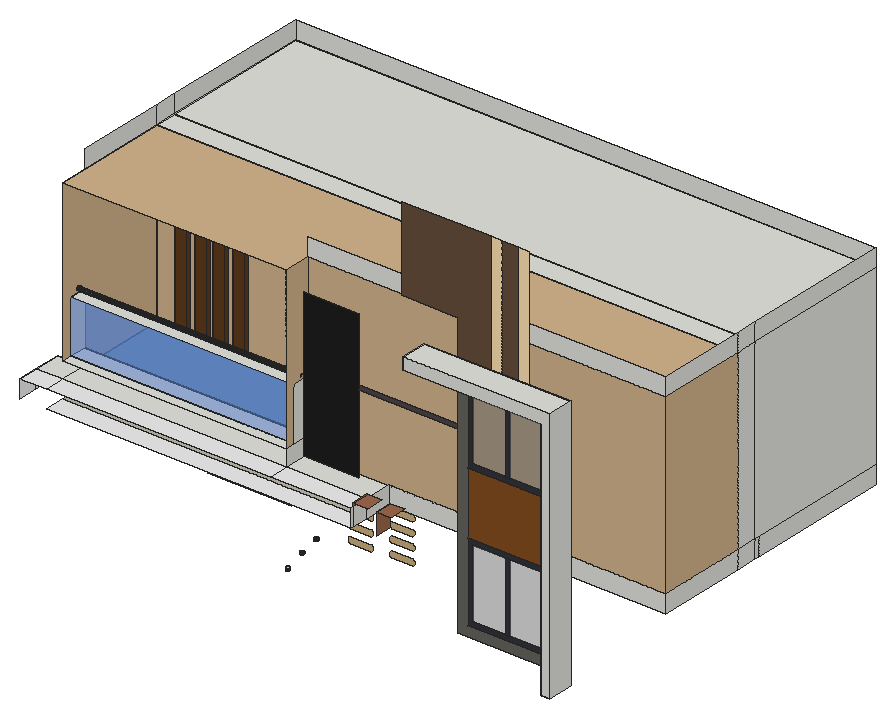
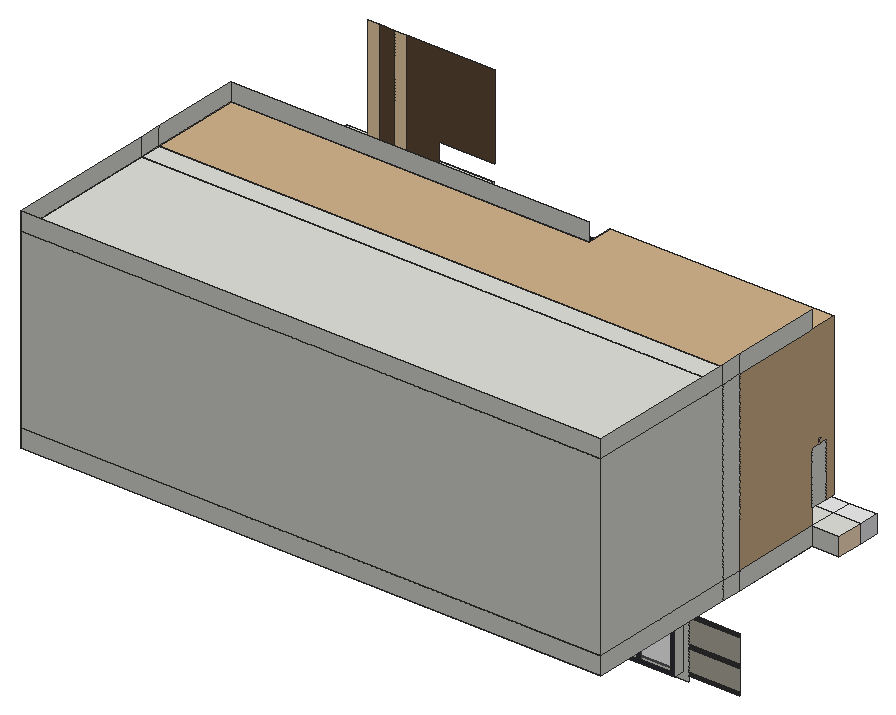
# SketchUp Ruby script. Lengths in inches.
U = 1.inch
M = Sketchup.active_model
def pt(a) = Geom::Point3d.new(a.map { |v| v * U })
def face(e, loops, mat)
  f = e.add_face(loops[0].map { |a| pt(a) })
  loops[1..].each { |l| e.add_face(l.map { |a| pt(a) }).erase! }
  f.material = f.back_material = mat if mat
  f
end
# faces: each face lists its corners as indices into pts; further lists are holes
def faces(e, pts, list, mat = nil) = list.each { |f| face(e, (f[0].is_a?(Array) ? f : [f]).map { |l| l.map { |i| pts[i] } }, mat) }
# xy, xz, yz: faces in a plane at the given z, y or x. An outline is a flat list of corners, or four numbers for a rectangle; further outlines are holes
def ring(l) = l.size == 4 ? [[l[0], l[1]], [l[2], l[1]], [l[2], l[3]], [l[0], l[3]]] : l.each_slice(2).to_a
def flat(e, list, mat, &to3) = list.each { |f| face(e, (f[0].is_a?(Array) ? f : [f]).map { |l| ring(l).map { |u, v| to3.(u, v) } }, mat) }
def xy(e, z, list, mat = nil) = flat(e, list, mat) { |x, y| [x, y, z] }
def xz(e, y, list, mat = nil) = flat(e, list, mat) { |x, z| [x, y, z] }
def yz(e, x, list, mat = nil) = flat(e, list, mat) { |y, z| [x, y, z] }
def lines(e, pts, list) = list.each { |a, b| e.add_line(pt(pts[a]), pt(pts[b])) }
# prism: a flat outline (further loops are holes) pulled along v
def prism(e, loops, v, mat = nil)
  f = face(e, loops, mat); d = Geom::Vector3d.new(v.map { |x| x * U })
  f.pushpull(f.normal.samedirection?(d) ? d.length : -d.length)
end
def box(e, o, s, mat = nil) = prism(e, [[o, [o[0] + s[0], o[1], o[2]], [o[0] + s[0], o[1] + s[1], o[2]], [o[0], o[1] + s[1], o[2]]]], [0, 0, s[2]], mat)
def at(x, y, z, deg = 0) = Geom::Transformation.translation(pt([x, y, z])) * Geom::Transformation.rotation(ORIGIN, Z_AXIS, deg.degrees)
def axes(o, x, y, z) = Geom::Transformation.new([*x, 0, *y, 0, *z, 0, *pt(o).to_a, 1])
def part(name) = M.definitions.add(name)
# library, detail: a bought-in or finely detailed component or shape, given as its bounding box
def library(name, o, s) = part(name).tap { |d| box(d.entities, o, s) }
def detail(e, o, s) = box(e.add_group.entities, o, s)
def put(e, d, t, mat = nil) = e.add_instance(d, t).tap { |i| i.material = mat if mat }
def group(e, t, mat = nil) = e.add_group.tap { |g| g.transformation = t; g.material = mat if mat }.entities
root = M.entities
M.materials.add("[0012_Bisque]").color = [255, 228, 196]
M.materials.add("[0035_Tan]").color = [210, 180, 140]
M.materials.add("[Asphalt New]").color = [79, 70, 73]
M.materials.add("[Blacktop New]").color = [30, 30, 30]
M.materials.add("[Blinds Vertical Pattern]").color = [237, 237, 239]
M.materials.add("[Carrera Marble]").color = [207, 207, 207]
M.materials.add("[Cladding Siding Tan]").color = [102, 79, 59]
M.materials.add("[Color M07]").color = [58, 58, 58]
M.materials.add("[Concrete Pavers Block Multi]").color = [124, 140, 145]
M.materials.add("[Formica Beige]").color = [255, 225, 180]
M.materials.add("[Formica Graystone]").color = [91, 89, 83]
M.materials.add("[Formica Graystone]1").color = [188, 184, 170]
M.materials.add("[Formica Graystone]2").color = [102, 99, 92]
M.materials.add("[Formica Laminate Dark]").color = [50, 53, 60]
M.materials.add("[Formica Speckled Grey]").color = [94, 105, 111]
M.materials.add("[Quartz Light Grey]").color = [251, 251, 252]
M.materials.add("[Translucent Glass Blue]").color = [106, 158, 252]
M.materials["[Translucent Glass Blue]"].alpha = 0.5
M.materials.add("[Translucent Glass Gray]").color = [128, 128, 128]
M.materials["[Translucent Glass Gray]"].alpha = 0.5
M.materials.add("[Wood Bamboo]").color = [130, 77, 31]
M.materials.add("[Wood Floor Light]").color = [204, 176, 127]
M.materials.add("[Wood Floor Parquet]").color = [96, 59, 26]
M.materials.add("[Wood Veneer 02]").color = [155, 104, 74]
prism(root,[[[158.39,214.66,43.5],[158.09,214.43,43.5],[157.74,214.28,43.5],[157.37,214.23,43.5],[157,214.28,43.5],[156.65,214.43,43.5],[156.35,214.66,43.5],[156.125,214.95,43.5],[155.98,215.3,43.5],[155.93,215.67,43.5],[155.98,216.04,43.5],[156.125,216.39,43.5],[156.35,216.6875,43.5],[156.65,216.92,43.5],[157,217.0625,43.5],[157.37,217.11,43.5],[157.74,217.0625,43.5],[158.09,216.92,43.5],[158.39,216.6875,43.5],[158.62,216.39,43.5],[158.76,216.04,43.5],[158.81,215.67,43.5],[158.76,215.3,43.5],[158.62,214.95,43.5]]],[0,0,1.5625])
prism(root,[[[157.57,229.04,47.875],[157.28,228.81,47.875],[156.93,228.66,47.875],[156.56,228.62,47.875],[156.1875,228.66,47.875],[155.84,228.81,47.875],[155.54,229.04,47.875],[155.3125,229.33,47.875],[155.17,229.68,47.875],[155.12,230.05,47.875],[155.17,230.43,47.875],[155.3125,230.77,47.875],[155.54,231.07,47.875],[155.84,231.3,47.875],[156.1875,231.44,47.875],[156.56,231.49,47.875],[156.93,231.44,47.875],[157.28,231.3,47.875],[157.57,231.07,47.875],[157.8,230.77,47.875],[157.95,230.43,47.875],[158,230.05,47.875],[157.95,229.68,47.875],[157.8,229.33,47.875]]],[0,0,1.3125])
prism(root,[[[158.3,241.66,51.6875],[158.01,241.43,51.6875],[157.66,241.29,51.6875],[157.29,241.24,51.6875],[156.92,241.29,51.6875],[156.57,241.43,51.6875],[156.27,241.66,51.6875],[156.04,241.96,51.6875],[155.9,242.31,51.6875],[155.85,242.68,51.6875],[155.9,243.05,51.6875],[156.04,243.4,51.6875],[156.27,243.7,51.6875],[156.57,243.92,51.6875],[156.92,244.07,51.6875],[157.29,244.12,51.6875],[157.66,244.07,51.6875],[158.01,243.92,51.6875],[158.3,243.7,51.6875],[158.53,243.4,51.6875],[158.68,243.05,51.6875],[158.72,242.68,51.6875],[158.68,242.31,51.6875],[158.53,241.96,51.6875]]],[0,0,1.3125])
xy(root,58.39,[[63.57,263.11,117.79,270.68]])
xy(root,69.56,[[397.29,154.7,397.98,174.45],[397.98,154.7,404.1,174.45]])
xy(root,104.92,[[63.57,263.11,117.79,270.68]])
xy(root,129,[[20.26,263.11,459.74,279.66],[20.26,279.66,459.74,394.19]])
xy(root,129,[[20.26,159.45,250.29,174.45]],"[Blinds Vertical Pattern]")
xy(root,129,[[20.26,174.45,20.26,263.11,459.74,263.11,459.74,194.72,250.29,194.72,250.29,174.45]],"[Formica Graystone]1")
xy(root,142.5625,[[0,174.45,20.26,194.72],[20.26,174.45,189.35,194.72],[189.35,174.45,250.29,194.72],[36.54,259.86,45.41,263.11],[51.85,259.86,60.73,263.11],
  [65.48,259.86,74.35,263.11],[80.48,259.86,89.35,263.11],[20.26,263.11,459.74,279.66],[20.26,279.66,459.74,394.19]])
xy(root,142.5625,[[0,159.45,20.26,174.45],[20.26,159.45,189.35,174.45],[189.35,159.45,250.29,174.45]],"[Blinds Vertical Pattern]")
xy(root,142.5625,[[20.26,194.72,459.74,194.72,459.74,263.11,89.35,263.11,89.35,259.86,80.48,259.86,80.48,263.11,74.35,263.11,74.35,259.86,65.48,259.86,65.48,263.11,60.73,263.11,60.73,259.86,51.85,259.86,51.85,263.11,45.41,263.11,45.41,259.86,36.54,259.86,36.54,263.11,20.26,263.11]],"[Concrete Pavers Block Multi]")
xy(root,145.3125,[[250.29,161.27,261.4375,174.45],[267.85,161.27,279,174.45]],"[Wood Veneer 02]")
xy(root,155,[[20.26,174.45,189.35,181.58],[20.26,181.58,189.35,194.72]])
xy(root,195.0625,[[20.26,181.58,189.35,194.72]])
xy(root,246.125,[[36.54,259.86,45.41,263.11],[51.85,259.86,60.73,263.11],[65.48,259.86,74.35,263.11],[80.48,259.86,89.35,263.11]],"[Wood Floor Parquet]")
xy(root,253.38,[[293.48,154.7,397.29,174.45]])
xy(root,262.44,[[293.48,154.7,404.1,174.45]])
xy(root,275.9375,[[20.26,263.11,459.74,279.66],[20.26,279.66,459.74,394.19]])
xy(root,275.9375,[[20.26,174.45,20.26,263.11,459.74,263.11,459.74,194.72,189.35,194.72,189.35,174.45]],"[0035_Tan]")
xz(root,154.7,[[397.29,69.56,404.1,69.56,404.1,262.44,293.48,262.44,293.48,253.38,397.29,253.38]])
xz(root,174.45,[[397.29,69.56,397.29,253.38,293.48,253.38,293.48,262.44,404.1,262.44,404.1,69.56]])
xz(root,174.45,[[244.42,213.94,319.23,217.18]],"[Asphalt New]")
xz(root,174.45,[[202.17,154.2,244.42,265.33]],"[Blacktop New]")
xz(root,174.45,[[319.23,262.44,343.68,262.44,343.68,352.96,276.43,352.96,276.43,289.4375,319.23,289.4375],[351.89,262.44,364.49,352.96]],"[Cladding Siding Tan]")
xz(root,174.45,[[343.68,262.44,351.89,352.96],[364.49,262.44,372.71,352.96]],"[Formica Beige]")
xz(root,174.45,[[[319.23,75.51,397.29,253.38],[326.77,83.05,389.74,245.84]]],"[Formica Graystone]2")
xz(root,174.45,[[[326.77,83.05,389.74,142.71],[330.47,86.75,386.05,139.01]],[355.2,86.75,358.26,139.01],[[326.77,190.14,389.74,245.84],[330.47,193.84,386.05,242.14]],[355.2,193.84,358.26,242.14]],"[Formica Laminate Dark]")
xz(root,174.45,[[330.47,86.75,355.2,139.01],[358.26,86.75,386.05,139.01],[330.47,193.84,355.2,242.14],[358.26,193.84,386.05,242.14]],"[Translucent Glass Gray]")
xz(root,174.45,[[326.77,142.71,389.74,190.14]],"[Wood Bamboo]")
xz(root,181.58,[[20.26,155,189.35,195.0625]],"[Translucent Glass Blue]")
xz(root,194.72,[[0,129,20.26,142.5625],[250.29,129,459.74,142.5625],[20.26,142.5625,189.35,155],[189.35,275.9375,459.74,289.4375]])
xz(root,194.72,[[189.35,142.5625,459.74,275.9375]],"[0035_Tan]")
xz(root,194.72,[[20.26,155,189.35,195.0625]],"[Translucent Glass Blue]")
xz(root,259.86,[[36.54,142.5625,45.41,246.125],[51.85,142.5625,60.73,246.125],[65.48,142.5625,74.35,246.125],[80.48,142.5625,89.35,246.125]],"[Wood Floor Parquet]")
xz(root,263.11,[[[58.93,53.75,122.43,109.5625],[63.57,58.39,117.79,104.92]],[20.26,129,459.74,142.5625],[36.54,142.5625,45.41,246.125],[51.85,142.5625,60.73,246.125],[65.48,142.5625,74.35,246.125],
  [80.48,142.5625,89.35,246.125]])
xz(root,263.11,[[20.26,142.5625,36.54,142.5625,36.54,246.125,45.41,246.125,45.41,142.5625,51.85,142.5625,51.85,246.125,60.73,246.125,60.73,142.5625,65.48,142.5625,65.48,246.125,74.35,246.125,74.35,142.5625,80.48,142.5625,80.48,246.125,89.35,246.125,89.35,142.5625,117.84,142.5625,117.84,253.1875,178.78,253.1875,178.78,142.5625,459.74,142.5625,459.74,275.9375,20.26,275.9375]],"[0035_Tan]")
xz(root,263.11,[[[121.46,146.18,146.67,249.57],[124.2,148.92,143.93,246.83]],[[149.4,146.18,175.16,249.57],[152.14,148.92,172.42,246.83]]],"[Carrera Marble]")
xz(root,263.11,[[20.26,57.76,58.93,60.64],[122.43,58.93,161.07,62.05],[20.26,76.19,58.93,79.08],[122.43,77.79,161.07,80.56],[20.26,97.13,58.93,100.02],
  [122.43,99.46,161.07,102.34]],"[Color M07]")
xz(root,263.11,[[20.26,60.64,58.93,76.19],[122.43,62.05,161.07,77.79],[20.26,79.08,58.93,97.13],[122.43,80.56,161.07,99.46],[124.2,148.92,132.28,163.16],
  [134.24,148.92,143.93,163.16],[152.14,148.92,160.32,163.5],[162.28,148.92,172.42,163.5],[124.2,165.34,132.28,177.39],[134.24,165.34,143.93,177.39],
  [152.14,165.6875,160.32,178.08],[162.28,165.6875,172.42,178.08],[124.2,179.58,132.28,191.95],[134.24,179.58,143.93,191.95],[152.14,180.27,160.32,192.83],
  [162.28,180.27,172.42,192.83],[124.2,194.14,132.28,206.27],[134.24,194.14,143.93,206.27],[152.14,195.02,160.32,208.27],[162.28,195.02,172.42,208.27],
  [124.2,208.45,132.28,220.33],[134.24,208.45,143.93,220.33],[152.14,210.45,160.32,220.52],[162.28,210.45,172.42,220.52],[124.2,222.52,132.28,232.2],
  [134.24,222.52,143.93,232.2],[152.14,222.7,160.32,232.2],[162.28,222.7,172.42,232.2],[124.2,234.39,132.28,246.83],[134.24,234.39,143.93,246.83],
  [152.14,234.39,160.32,246.83],[162.28,234.39,172.42,246.83]],"[Formica Graystone]1")
xz(root,263.11,[[191.9,69.69,194.09,89.19],[186.95,69.82,189.63,89.25]],"[Formica Laminate Dark]")
xz(root,263.11,[[132.28,148.92,134.24,148.92,134.24,163.16,143.93,163.16,143.93,165.34,134.24,165.34,134.24,177.39,143.93,177.39,143.93,179.58,134.24,179.58,134.24,191.95,143.93,191.95,143.93,194.14,134.24,194.14,134.24,206.27,143.93,206.27,143.93,208.45,134.24,208.45,134.24,220.33,143.93,220.33,143.93,222.52,134.24,222.52,134.24,232.2,143.93,232.2,143.93,234.39,134.24,234.39,134.24,246.83,132.28,246.83,132.28,234.39,124.2,234.39,124.2,232.2,132.28,232.2,132.28,222.52,124.2,222.52,124.2,220.33,132.28,220.33,132.28,208.45,124.2,208.45,124.2,206.27,132.28,206.27,132.28,194.14,124.2,194.14,124.2,191.95,132.28,191.95,132.28,179.58,124.2,179.58,124.2,177.39,132.28,177.39,132.28,165.34,124.2,165.34,124.2,163.16,132.28,163.16],[160.32,148.92,162.28,148.92,162.28,163.5,172.42,163.5,172.42,165.6875,162.28,165.6875,162.28,178.08,172.42,178.08,172.42,180.27,162.28,180.27,162.28,192.83,172.42,192.83,172.42,195.02,162.28,195.02,162.28,208.27,172.42,208.27,172.42,210.45,162.28,210.45,162.28,220.52,172.42,220.52,172.42,222.7,162.28,222.7,162.28,232.2,160.32,232.2,160.32,222.7,152.14,222.7,152.14,220.52,160.32,220.52,160.32,210.45,152.14,210.45,152.14,208.27,160.32,208.27,160.32,195.02,152.14,195.02,152.14,192.83,160.32,192.83,160.32,180.27,152.14,180.27,152.14,178.08,160.32,178.08,160.32,165.6875,152.14,165.6875,152.14,163.5,160.32,163.5],[152.14,232.2,172.42,234.39],[160.32,234.39,162.28,246.83]],"[Formica Speckled Grey]")
xz(root,263.11,[[[117.84,142.5625,178.78,253.1875],[121.46,146.18,175.16,249.57]],[146.67,146.18,149.4,249.57]],"[Quartz Light Grey]")
xz(root,263.11,[[166.93,43.73,182.32,43.73,182.8,43.94,183.23,44.24,183.59,44.63,183.85,45.09,184.02,45.58,184.07,46.11,184.02,46.63,183.85,47.13,183.59,47.58,183.23,47.97,182.8,48.27,182.32,48.48,166.93,48.48,166.48,48.26,166.07,47.94,165.74,47.55,165.49,47.1,165.34,46.62,165.29,46.11,165.34,45.6,165.49,45.11,165.74,44.66,166.07,44.27,166.48,43.96],[198.25,44.86,213.63,44.86,214.12,45.06,214.54,45.37,214.9,45.76,215.16,46.21,215.33,46.71,215.38,47.23,215.33,47.75,215.16,48.25,214.9,48.71,214.54,49.09,214.12,49.4,213.63,49.61,198.25,49.61,197.79,49.38,197.38,49.07,197.05,48.68,196.8,48.23,196.65,47.74,196.6,47.23,196.65,46.72,196.8,46.23,197.05,45.79,197.38,45.4,197.79,45.08],[166.93,53.98,182.32,53.98,182.8,54.19,183.23,54.49,183.59,54.88,183.85,55.34,184.02,55.83,184.07,56.36,184.02,56.88,183.85,57.38,183.59,57.83,183.23,58.22,182.8,58.52,182.32,58.73,166.93,58.73,166.48,58.51,166.07,58.19,165.74,57.8,165.49,57.35,165.34,56.87,165.29,56.36,165.34,55.85,165.49,55.36,165.74,54.91,166.07,54.52,166.48,54.21],[198.25,54.92,213.63,54.92,214.12,55.13,214.54,55.43,214.9,55.82,215.16,56.27,215.33,56.77,215.38,57.29,215.33,57.82,215.16,58.32,214.9,58.77,214.54,59.16,214.12,59.46,213.63,59.67,198.25,59.67,197.79,59.44,197.38,59.13,197.05,58.74,196.8,58.29,196.65,57.8,196.6,57.29,196.65,56.79,196.8,56.3,197.05,55.85,197.38,55.46,197.79,55.15],[166.93,64.23,182.32,64.23,182.8,64.44,183.23,64.74,183.59,65.13,183.85,65.59,184.02,66.08,184.07,66.61,184.02,67.13,183.85,67.63,183.59,68.08,183.23,68.47,182.8,68.77,182.32,68.98,166.93,68.98,166.48,68.76,166.07,68.44,165.74,68.05,165.49,67.6,165.34,67.12,165.29,66.61,165.34,66.1,165.49,65.61,165.74,65.16,166.07,64.77,166.48,64.46],
  [198.25,64.98,213.63,64.98,214.12,65.19,214.54,65.49,214.9,65.88,215.16,66.34,215.33,66.83,215.38,67.36,215.33,67.88,215.16,68.38,214.9,68.83,214.54,69.22,214.12,69.52,213.63,69.73,198.25,69.73,197.79,69.51,197.38,69.19,197.05,68.8,196.8,68.35,196.65,67.87,196.6,67.36,196.65,66.85,196.8,66.36,197.05,65.91,197.38,65.52,197.79,65.21],[166.93,74.48,182.32,74.48,182.8,74.69,183.23,74.99,183.59,75.38,183.85,75.84,184.02,76.33,184.07,76.86,184.02,77.38,183.85,77.88,183.59,78.33,183.23,78.72,182.8,79.02,182.32,79.23,166.93,79.23,166.48,79.01,166.07,78.69,165.74,78.3,165.49,77.85,165.34,77.37,165.29,76.86,165.34,76.35,165.49,75.86,165.74,75.41,166.07,75.02,166.48,74.71],[198.25,75.04,213.63,75.04,214.12,75.25,214.54,75.56,214.9,75.94,215.16,76.4,215.33,76.9,215.38,77.42,215.33,77.94,215.16,78.44,214.9,78.89,214.54,79.28,214.12,79.59,213.63,79.79,198.25,79.79,197.79,79.57,197.38,79.25,197.05,78.86,196.8,78.42,196.65,77.93,196.6,77.42,196.65,76.91,196.8,76.42,197.05,75.97,197.38,75.59,197.79,75.27],[166.93,84.73,182.32,84.73,182.8,84.94,183.23,85.24,183.59,85.63,183.85,86.09,184.02,86.58,184.07,87.11,184.02,87.63,183.85,88.13,183.59,88.58,183.23,88.97,182.8,89.27,182.32,89.48,166.93,89.48,166.48,89.26,166.07,88.94,165.74,88.55,165.49,88.1,165.34,87.62,165.29,87.11,165.34,86.6,165.49,86.11,165.74,85.66,166.07,85.27,166.48,84.96],[198.25,85.11,213.63,85.11,214.12,85.31,214.54,85.62,214.9,86.01,215.16,86.46,215.33,86.96,215.38,87.48,215.33,88,215.16,88.5,214.9,88.96,214.54,89.34,214.12,89.65,213.63,89.86,198.25,89.86,197.79,89.63,197.38,89.32,197.05,88.93,196.8,88.48,196.65,87.99,196.6,87.48,196.65,86.97,196.8,86.48,197.05,86.04,197.38,85.65,197.79,85.33],
  [166.93,94.98,182.32,94.98,182.8,95.19,183.23,95.49,183.59,95.88,183.85,96.34,184.02,96.83,184.07,97.36,184.02,97.88,183.85,98.38,183.59,98.83,183.23,99.22,182.8,99.52,182.32,99.73,166.93,99.73,166.48,99.51,166.07,99.19,165.74,98.8,165.49,98.35,165.34,97.87,165.29,97.36,165.34,96.85,165.49,96.36,165.74,95.91,166.07,95.52,166.48,95.21],[198.25,95.17,213.63,95.17,214.12,95.38,214.54,95.68,214.9,96.07,215.16,96.52,215.33,97.02,215.38,97.54,215.33,98.07,215.16,98.57,214.9,99.02,214.54,99.41,214.12,99.71,213.63,99.92,198.25,99.92,197.79,99.69,197.38,99.38,197.05,98.99,196.8,98.54,196.65,98.05,196.6,97.54,196.65,97.04,196.8,96.55,197.05,96.1,197.38,95.71,197.79,95.4],[166.93,105.23,182.32,105.23,182.8,105.44,183.23,105.74,183.59,106.13,183.85,106.59,184.02,107.08,184.07,107.61,184.02,108.13,183.85,108.63,183.59,109.08,183.23,109.47,182.8,109.77,182.32,109.98,166.93,109.98,166.48,109.76,166.07,109.44,165.74,109.05,165.49,108.6,165.34,108.12,165.29,107.61,165.34,107.1,165.49,106.61,165.74,106.16,166.07,105.77,166.48,105.46],[198.25,105.23,213.63,105.23,214.12,105.44,214.54,105.74,214.9,106.13,215.16,106.59,215.33,107.08,215.38,107.61,215.33,108.13,215.16,108.63,214.9,109.08,214.54,109.47,214.12,109.77,213.63,109.98,198.25,109.98,197.79,109.76,197.38,109.44,197.05,109.05,196.8,108.6,196.65,108.12,196.6,107.61,196.65,107.1,196.8,106.61,197.05,106.16,197.38,105.77,197.79,105.46]],"[Wood Floor Light]")
xz(root,270.68,[[[63.57,58.39,117.79,104.92],[66.15,60.97,115.21,102.34]],[89.12,60.97,92.35,102.34]],"[Formica Laminate Dark]")
xz(root,270.68,[[66.15,60.97,89.12,102.34],[92.35,60.97,115.21,102.34]],"[Translucent Glass Gray]")
xz(root,279.66,[[20.26,129,459.74,142.5625],[20.26,142.5625,459.74,275.9375]])
xz(root,394.19,[[20.26,129,459.74,142.5625],[20.26,142.5625,459.74,275.9375],[20.26,275.9375,459.74,289.4375]])
yz(root,0,[[174.45,129,194.72,142.5625]],"[0012_Bisque]")
yz(root,0,[[159.45,129,174.45,142.5625]],"[Blinds Vertical Pattern]")
yz(root,20.26,[[194.72,129,263.11,142.5625],[263.11,129,279.66,142.5625],[279.66,129,394.19,142.5625],[263.11,142.5625,279.66,275.9375],[279.66,142.5625,394.19,275.9375],
  [181.58,155,194.72,195.0625],[188.18,197.1,187.81,197.15,187.46,197.29,187.16,197.52,186.93,197.82,186.79,198.17,186.74,198.54,186.79,198.91,186.93,199.26,187.16,199.56,187.46,199.78,187.81,199.93,188.18,199.98,188.55,199.93,188.9,199.78,189.19,199.56,189.42,199.26,189.57,198.91,189.61,198.54,189.57,198.17,189.42,197.82,189.19,197.52,188.9,197.29,188.55,197.15],[194.72,275.9375,263.11,289.4375],[263.11,275.9375,279.66,289.4375],[279.66,275.9375,394.19,289.4375]])
yz(root,20.26,[[[194.72,142.5625,263.11,142.5625,263.11,275.9375,174.45,275.9375,174.45,155,181.58,155,181.58,195.0625,194.72,195.0625],[188.18,197.1,187.81,197.15,187.46,197.29,187.16,197.52,186.93,197.82,186.79,198.17,186.74,198.54,186.79,198.91,186.93,199.26,187.16,199.56,187.46,199.78,187.81,199.93,188.18,199.98,188.55,199.93,188.9,199.78,189.19,199.56,189.42,199.26,189.57,198.91,189.61,198.54,189.57,198.17,189.42,197.82,189.19,197.52,188.9,197.29,188.55,197.15]]],"[0035_Tan]")
yz(root,36.54,[[259.86,142.5625,263.11,246.125]],"[Wood Floor Parquet]")
yz(root,45.41,[[259.86,142.5625,263.11,246.125]],"[Wood Floor Parquet]")
yz(root,51.85,[[259.86,142.5625,263.11,246.125]],"[Wood Floor Parquet]")
yz(root,60.73,[[259.86,142.5625,263.11,246.125]],"[Wood Floor Parquet]")
yz(root,63.57,[[263.11,58.39,270.68,104.92]])
yz(root,65.48,[[259.86,142.5625,263.11,246.125]],"[Wood Floor Parquet]")
yz(root,74.35,[[259.86,142.5625,263.11,246.125]],"[Wood Floor Parquet]")
yz(root,80.48,[[259.86,142.5625,263.11,246.125]],"[Wood Floor Parquet]")
yz(root,89.35,[[259.86,142.5625,263.11,246.125]],"[Wood Floor Parquet]")
yz(root,117.79,[[263.11,58.39,270.68,104.92]])
yz(root,189.35,[[174.45,142.5625,194.72,155],[181.58,155,194.72,195.0625]])
yz(root,189.35,[[[174.45,155,174.45,275.9375,194.72,275.9375,194.72,195.0625,181.58,195.0625,181.58,155],[188.18,197.1,188.55,197.15,188.9,197.29,189.19,197.52,189.42,197.82,189.57,198.17,189.61,198.54,189.57,198.91,189.42,199.26,189.19,199.56,188.9,199.78,188.55,199.93,188.18,199.98,187.81,199.93,187.46,199.78,187.16,199.56,186.93,199.26,186.79,198.91,186.74,198.54,186.79,198.17,186.93,197.82,187.16,197.52,187.46,197.29,187.81,197.15]]],"[0035_Tan]")
yz(root,250.29,[[159.45,129,161.27,142.5625],[161.27,129,174.45,142.5625],[174.45,129,194.72,142.5625]])
yz(root,250.29,[[161.27,142.5625,174.45,145.3125]],"[Wood Veneer 02]")
yz(root,267.85,[[161.27,129,174.45,145.3125]],"[Wood Veneer 02]")
yz(root,293.48,[[154.7,253.38,174.45,262.44]])
yz(root,397.29,[[154.7,69.56,174.45,253.38]])
yz(root,404.1,[[154.7,69.56,174.45,262.44]])
yz(root,459.74,[[194.72,129,263.11,142.5625],[263.11,129,279.66,142.5625],[279.66,129,283.36,142.5625],[283.36,129,394.19,142.5625],[263.11,142.5625,279.66,275.9375],
  [279.66,142.5625,394.19,275.9375],[194.72,275.9375,263.11,289.4375],[263.11,275.9375,279.66,289.4375],[279.66,275.9375,394.19,289.4375]])
yz(root,459.74,[[194.72,142.5625,263.11,275.9375]],"[0035_Tan]")
p = [[20.26,187.81,197.15],[20.26,188.18,197.1],[189.35,188.18,197.1],[189.35,187.81,197.15],[20.26,188.55,197.15],[189.35,188.55,197.15],
  [20.26,187.46,197.29],[189.35,187.46,197.29],[20.26,188.9,197.29],[189.35,188.9,197.29],[20.26,187.16,197.52],[189.35,187.16,197.52],
  [20.26,189.19,197.52],[189.35,189.19,197.52],[20.26,186.93,197.82],[189.35,186.93,197.82],[20.26,189.42,197.82],[189.35,189.42,197.82],
  [20.26,186.79,198.17],[189.35,186.79,198.17],[20.26,189.57,198.17],[189.35,189.57,198.17],[20.26,186.74,198.54],[189.35,186.74,198.54],
  [20.26,189.61,198.54],[189.35,189.61,198.54],[20.26,186.79,198.91],[189.35,186.79,198.91],[20.26,189.57,198.91],[189.35,189.57,198.91],
  [20.26,186.93,199.26],[189.35,186.93,199.26],[20.26,189.42,199.26],[189.35,189.42,199.26],[20.26,187.16,199.56],[189.35,187.16,199.56],
  [20.26,189.19,199.56],[189.35,189.19,199.56],[20.26,187.46,199.78],[189.35,187.46,199.78],[20.26,188.9,199.78],[189.35,188.9,199.78],
  [20.26,187.81,199.93],[189.35,187.81,199.93],[20.26,188.55,199.93],[189.35,188.55,199.93],[20.26,188.18,199.98],[189.35,188.18,199.98]]
faces(root,p,[[0,1,2,3],[1,4,5,2],[6,0,3,7],[4,8,9,5],[10,6,7,11],[8,12,13,9],[14,10,11,15],[12,16,17,13],
  [18,14,15,19],[16,20,21,17],[22,18,19,23],[20,24,25,21],[26,22,23,27],[24,28,29,25],[30,26,27,31],[28,32,33,29],
  [34,30,31,35],[32,36,37,33],[38,34,35,39],[36,40,41,37],[42,38,39,43],[40,44,45,41],[46,42,43,47],[44,46,47,45]],"[Formica Graystone]")
